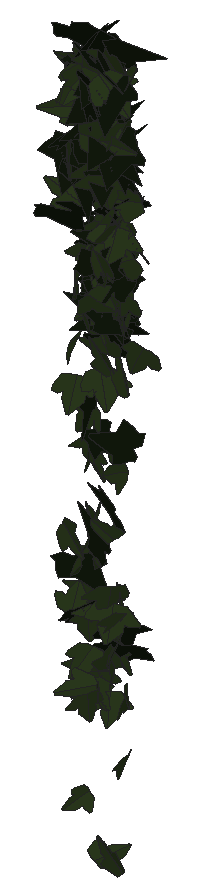
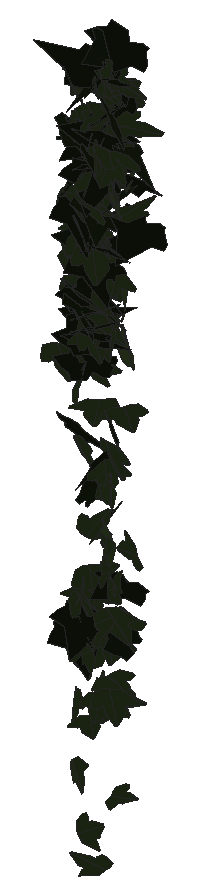
# SketchUp Ruby script. Lengths in inches.
U = 1.inch
M = Sketchup.active_model
def pt(a) = Geom::Point3d.new(a.map { |v| v * U })
def face(e, loops, mat)
  f = e.add_face(loops[0].map { |a| pt(a) })
  loops[1..].each { |l| e.add_face(l.map { |a| pt(a) }).erase! }
  f.material = f.back_material = mat if mat
  f
end
# faces: each face lists its corners as indices into pts; further lists are holes
def faces(e, pts, list, mat = nil) = list.each { |f| face(e, (f[0].is_a?(Array) ? f : [f]).map { |l| l.map { |i| pts[i] } }, mat) }
# xy, xz, yz: faces in a plane at the given z, y or x. An outline is a flat list of corners, or four numbers for a rectangle; further outlines are holes
def ring(l) = l.size == 4 ? [[l[0], l[1]], [l[2], l[1]], [l[2], l[3]], [l[0], l[3]]] : l.each_slice(2).to_a
def flat(e, list, mat, &to3) = list.each { |f| face(e, (f[0].is_a?(Array) ? f : [f]).map { |l| ring(l).map { |u, v| to3.(u, v) } }, mat) }
def xy(e, z, list, mat = nil) = flat(e, list, mat) { |x, y| [x, y, z] }
def xz(e, y, list, mat = nil) = flat(e, list, mat) { |x, z| [x, y, z] }
def yz(e, x, list, mat = nil) = flat(e, list, mat) { |y, z| [x, y, z] }
def lines(e, pts, list) = list.each { |a, b| e.add_line(pt(pts[a]), pt(pts[b])) }
# prism: a flat outline (further loops are holes) pulled along v
def prism(e, loops, v, mat = nil)
  f = face(e, loops, mat); d = Geom::Vector3d.new(v.map { |x| x * U })
  f.pushpull(f.normal.samedirection?(d) ? d.length : -d.length)
end
def box(e, o, s, mat = nil) = prism(e, [[o, [o[0] + s[0], o[1], o[2]], [o[0] + s[0], o[1] + s[1], o[2]], [o[0], o[1] + s[1], o[2]]]], [0, 0, s[2]], mat)
def at(x, y, z, deg = 0) = Geom::Transformation.translation(pt([x, y, z])) * Geom::Transformation.rotation(ORIGIN, Z_AXIS, deg.degrees)
def axes(o, x, y, z) = Geom::Transformation.new([*x, 0, *y, 0, *z, 0, *pt(o).to_a, 1])
def part(name) = M.definitions.add(name)
# library, detail: a bought-in or finely detailed component or shape, given as its bounding box
def library(name, o, s) = part(name).tap { |d| box(d.entities, o, s) }
def detail(e, o, s) = box(e.add_group.entities, o, s)
def put(e, d, t, mat = nil) = e.add_instance(d, t).tap { |i| i.material = mat if mat }
def group(e, t, mat = nil) = e.add_group.tap { |g| g.transformation = t; g.material = mat if mat }.entities
root = M.entities
M.materials.add("1026 AP 7946 SUNNY SIDE UP").color = [254, 231, 186]
M.materials.add("efeu1").color = [18, 25, 13]
M.materials.add("efeu2").color = [43, 57, 29]
c1 = part("ivyleaf_10")
p = [[0,0.5,-0.03],[-0.0625,2.02,-0.43],[-0.19,2.01,-0.46],[-0.54,1.05,-0.29],[-0.52,0.625,-0.18],[-0.83,0.76,-0.28],
  [-1.16,0.64,-0.33],[-1.15,0.33,-0.24],[-0.77,-0.39,0.02],[-0.3,-0.51,0.16],[0.04,-0.48,0.23],[-0.02,2.01,-0.4375],
  [-0.06,2.01,-0.43],[0.04,-0.49,0.23],[0.67,-0.49,0.14],[1.38,0.36,-0.2],[1.375,0.51,-0.24],[0.81,0.65,-0.19],
  [0.62,0.59,-0.15],[0.6,1.09,-0.28],[0.5,1.23,-0.31]]
faces(c1.entities,p,[[0,1,2,3,4,5,6,7,8,9,10],[11,12,0,13,14,15,16,17,18,19,20]],"efeu2")
c2 = part("ivyleaf_9")
p = [[1.54,2.16,1.25],[1.36,2.04,1.19],[-0.21,0.99,0.68],[-0.71,1.11,0.82],[-0.85,0.86,0.67],[-0.8,0.17,0.21],
  [-0.9,-0.01,0.1],[-0.67,-0.16,-0.02],[-0.08,-0.08,-0.05],[-0.03,-0.6,-0.4],[0.65,-0.88,-0.66],[0.83,-0.6,-0.49],
  [1.29,-0.42,-0.43],[1.8125,-0.07,-0.26],[1.21,0.44,0.15]]
faces(c2.entities,p,[[0,1,2,3,4,5,6,7,8,9,10,11,12,13,14]],"efeu1")
put(root,c1,axes([144.45,212.06,261.74],[0.01803,-0.18534,-0.18854],[0.09388,-0.17538,0.18688],[-0.39747,-0.04983,0.03559]),"1026 AP 7946 SUNNY SIDE UP")
put(root,c1,axes([144.87,211.93,255.18],[-0.1348,-0.22159,-0.03975],[0.06097,0.02477,-0.24305],[0.34804,-0.09016,0.02718]),"1026 AP 7946 SUNNY SIDE UP")
put(root,c1,axes([144.71,212.06,253.23],[0.088,0.07575,-0.18545],[-0.14235,-0.15637,-0.09747],[-0.27281,0.10602,-0.00896]),"1026 AP 7946 SUNNY SIDE UP")
put(root,c1,axes([144.34,212.09,265.43],[-0.07276,0.14566,-0.23472],[0.08159,-0.22293,-0.15841],[-0.41843,-0.0688,0.00993]),"1026 AP 7946 SUNNY SIDE UP")
put(root,c2,axes([145.21,212.11,266.96],[-0.32431,-0.1331,-0.196],[0.34711,-0.03636,-0.22143],[0.10998,-0.27772,0.1209]),"1026 AP 7946 SUNNY SIDE UP")
put(root,c1,axes([145.13,211.92,263.67],[-0.315,0.15747,0.02528],[-0.04992,-0.00227,-0.2616],[-0.24536,-0.20171,0.02078]),"1026 AP 7946 SUNNY SIDE UP")
put(root,c2,axes([145.16,211.98,258.11],[-0.04449,-0.23121,0.13442],[0.04104,0.12949,0.24055],[-0.41646,0.03746,0.00935]),"1026 AP 7946 SUNNY SIDE UP")
put(root,c1,axes([145.04,211.86,262.92],[-0.1515,-0.15169,-0.19123],[0.17748,0.14673,-0.18389],[0.33135,-0.14795,0.01106]),"1026 AP 7946 SUNNY SIDE UP")
put(root,c1,axes([145.5,211.92,252.2],[-0.20704,0.08706,-0.17581],[-0.21304,0.10493,0.16299],[0.21396,0.18873,-0.00784]),"1026 AP 7946 SUNNY SIDE UP")
put(root,c1,axes([144.92,211.94,265.875],[-0.00116,-0.00938,0.2927],[0.41626,0.10365,0.00484],[-0.16311,0.26459,0.01027]),"1026 AP 7946 SUNNY SIDE UP")
put(root,c2,axes([145.27,212.12,258.8],[0.15451,-0.24106,0.03262],[0.00824,0.03771,0.26769],[-0.3825,-0.09656,0.01894]),"1026 AP 7946 SUNNY SIDE UP")
put(root,c1,axes([145.125,211.91,263.71],[-0.02194,0.23657,0.10266],[-0.00865,0.09815,-0.24356],[-0.40272,-0.01499,-0.00036]),"1026 AP 7946 SUNNY SIDE UP")
put(root,c1,axes([144.45,212.09,264.51],[0.02544,0.20991,0.15199],[-0.10758,-0.13774,0.21053],[0.38771,-0.05199,0.04845]),"1026 AP 7946 SUNNY SIDE UP")
put(root,c1,axes([144.6,212.15,266.86],[0.14605,0.16517,-0.21623],[-0.18426,-0.1756,-0.19593],[-0.37868,0.14915,0.01194]),"1026 AP 7946 SUNNY SIDE UP")
put(root,c1,axes([144.54,212.14,266.875],[0.17303,0.19063,-0.17859],[-0.11346,-0.15939,-0.22727],[-0.39015,0.1309,-0.01312]),"1026 AP 7946 SUNNY SIDE UP")
put(root,c2,axes([145.09,211.89,263.4],[-0.12994,-0.02228,0.24889],[0.33848,0.11129,0.08703],[-0.17642,0.22994,-0.01633]),"1026 AP 7946 SUNNY SIDE UP")
put(root,c1,axes([145.28,212.06,256.92],[0.36629,0.11595,-0.02087],[-0.01282,-0.03038,-0.26715],[-0.18482,0.23191,-0.02284]),"1026 AP 7946 SUNNY SIDE UP")
put(root,c2,axes([144.22,211.9,264.32],[0.34278,0.1723,-0.00282],[0.01511,-0.01813,-0.28561],[-0.27057,0.21727,-0.01952]),"1026 AP 7946 SUNNY SIDE UP")
put(root,c1,axes([145.26,212.05,257.3],[-0.21369,-0.23241,0.00403],[0.00829,-0.00914,-0.27725],[0.36544,-0.13569,0.00865]),"1026 AP 7946 SUNNY SIDE UP")
put(root,c2,axes([144.92,211.9,266.41],[0.04695,-0.02726,0.29068],[-0.11428,0.27366,0.03674],[-0.43108,-0.07551,0.02192]),"1026 AP 7946 SUNNY SIDE UP")
put(root,c1,axes([144.24,212.14,258.07],[0.13555,-0.0311,0.23828],[0.33648,-0.08832,-0.09484],[0.14711,0.23067,-0.00262]),"1026 AP 7946 SUNNY SIDE UP")
put(root,c2,axes([145.24,212.2,266.0625],[-0.34855,-0.16205,-0.01746],[0.04188,-0.00937,-0.28191],[0.2526,-0.22205,0.02264]),"1026 AP 7946 SUNNY SIDE UP")
put(root,c1,axes([145.42,212.13,256.8125],[-0.07764,-0.24735,0.06803],[-0.02721,-0.06531,-0.26019],[0.40221,-0.05216,-0.00447]),"1026 AP 7946 SUNNY SIDE UP")
put(root,c1,axes([144.4,212.24,262.9],[-0.04091,0.05186,-0.26232],[0.0678,-0.25179,-0.05878],[-0.40339,-0.04758,0.01672]),"1026 AP 7946 SUNNY SIDE UP")
put(root,c1,axes([144.57,212.18,266.27],[0.12976,0.00512,-0.27205],[-0.37496,-0.11758,-0.0798],[-0.17867,0.25047,-0.03011]),"1026 AP 7946 SUNNY SIDE UP")
put(root,c2,axes([144.71,212.125,267.34],[0.28113,-0.21539,0.05224],[0.08571,-0.02193,-0.28712],[0.33768,0.18489,0.02938]),"1026 AP 7946 SUNNY SIDE UP")
put(root,c1,axes([145.22,211.98,266.99],[0.17671,0.24407,0.12792],[0.11107,0.10229,-0.27549],[-0.41499,0.1313,-0.01927]),"1026 AP 7946 SUNNY SIDE UP")
put(root,c1,axes([145.52,212.01,259.7],[0.16452,-0.14291,-0.17497],[-0.18773,0.12099,-0.18081],[0.29307,0.15773,-0.0176]),"1026 AP 7946 SUNNY SIDE UP")
put(root,c2,axes([144.5625,212.04,265.84],[-0.20079,0.24005,-0.04224],[0.00496,-0.04619,-0.27971],[-0.38325,-0.12636,0.01851]),"1026 AP 7946 SUNNY SIDE UP")
put(root,c1,axes([145.11,212.08,265.06],[-0.32834,-0.16825,-0.03101],[0.05736,0.00102,-0.27532],[0.2623,-0.21083,0.02139]),"1026 AP 7946 SUNNY SIDE UP")
put(root,c1,axes([145.14,212.2,258.25],[-0.15622,-0.12955,-0.14412],[-0.16373,-0.0943,0.16647],[-0.25013,0.14263,-0.01896]),"1026 AP 7946 SUNNY SIDE UP")
put(root,c2,axes([145.26,212.24,265.77],[-0.28645,-0.19422,-0.06174],[0.11708,0.00957,-0.27003],[0.29684,-0.1912,0.04693]),"1026 AP 7946 SUNNY SIDE UP")
put(root,c2,axes([144.42,212.29,264.92],[0.04612,-0.27459,0.10193],[0.01391,-0.10013,-0.28507],[0.45957,0.03059,-0.0016]),"1026 AP 7946 SUNNY SIDE UP")
put(root,c1,axes([145.375,212.19,266.09],[-0.01546,-0.29313,0.06983],[0.03207,-0.06998,-0.3017],[0.47259,-0.00484,0.02276]),"1026 AP 7946 SUNNY SIDE UP")
put(root,c1,axes([145.31,212.18,256.375],[0.18709,-0.22729,0.04707],[0.03074,-0.04279,-0.26454],[0.36365,0.12055,-0.00185]),"1026 AP 7946 SUNNY SIDE UP")
put(root,c1,axes([144.63,212.26,255.18],[-0.1137,0.00947,0.23017],[-0.13325,-0.2184,-0.02],[0.32531,-0.08615,0.07225]),"1026 AP 7946 SUNNY SIDE UP")
put(root,c2,axes([144.78,212.34,266.36],[-0.17899,-0.16344,0.19714],[-0.11589,-0.18023,-0.20381],[0.37953,-0.13211,0.03074]),"1026 AP 7946 SUNNY SIDE UP")
put(root,c1,axes([145.19,212.07,265.95],[0.07529,0.08139,0.30112],[-0.47619,0.00452,0.04992],[0.01345,-0.2957,0.08178]),"1026 AP 7946 SUNNY SIDE UP")
put(root,c2,axes([144.58,212.05,266.91],[0.42803,-0.06141,-0.13887],[-0.21558,0.00042,-0.28615],[0.08688,0.30361,-0.02585]),"1026 AP 7946 SUNNY SIDE UP")
put(root,c2,axes([144.375,212.25,265.36],[-0.34713,-0.11976,-0.11273],[0.19364,-0.00511,-0.25177],[0.16495,-0.24604,0.05832]),"1026 AP 7946 SUNNY SIDE UP")
put(root,c2,axes([144.99,212.07,265.83],[-0.07772,-0.11834,-0.26902],[0.19136,0.23051,-0.13034],[0.40711,-0.13095,0.00991]),"1026 AP 7946 SUNNY SIDE UP")
put(root,c2,axes([145.03,212.3125,266.1],[-0.01931,-0.02639,-0.26721],[-0.01289,-0.25935,0.02608],[-0.40952,0.0094,0.01178]),"1026 AP 7946 SUNNY SIDE UP")
put(root,c1,axes([145.1,212.3,255.68],[-0.05123,0.02836,0.25146],[0.23785,-0.19153,0.04263],[0.3042,0.15453,0.00901]),"1026 AP 7946 SUNNY SIDE UP")
put(root,c2,axes([144.49,212.03,267.78],[0.41426,0.11758,-0.00252],[0.01035,-0.02238,-0.29639],[-0.18465,0.26253,-0.02228]),"1026 AP 7946 SUNNY SIDE UP")
put(root,c1,axes([145.24,212.19,264.03],[0.3744,0.09825,-0.03775],[-0.04011,-0.03533,-0.26454],[-0.16026,0.23839,-0.02199]),"1026 AP 7946 SUNNY SIDE UP")
put(root,c1,axes([144.77,212.1,267.06],[0.04095,-0.0314,-0.28786],[-0.38408,0.13611,-0.03844],[0.21843,0.24521,-0.01363]),"1026 AP 7946 SUNNY SIDE UP")
put(root,c2,axes([144.86,212.3,265.38],[-0.19112,-0.24931,-0.07187],[0.08085,0.0507,-0.28443],[0.39836,-0.1299,0.02325]),"1026 AP 7946 SUNNY SIDE UP")
put(root,c1,axes([144.92,212.21,265.18],[-0.21788,-0.25791,-0.00189],[0.0244,-0.00792,-0.30113],[0.4048,-0.13834,0.01714]),"1026 AP 7946 SUNNY SIDE UP")
put(root,c1,axes([145.42,212.1875,262.89],[-0.35227,0.02531,0.08134],[-0.1277,-0.0232,-0.23028],[-0.02519,-0.23636,0.0299]),"1026 AP 7946 SUNNY SIDE UP")
put(root,c1,axes([144.8,212.34,255.27],[0.02106,-0.08763,-0.19104],[0.04436,-0.18278,0.09026],[-0.31873,-0.03123,-0.00006]),"1026 AP 7946 SUNNY SIDE UP")
put(root,c2,axes([145.28,212.06,262.98],[-0.3796,0.11924,-0.02877],[-0.02554,0.0315,0.27673],[0.19111,0.24105,-0.02016]),"1026 AP 7946 SUNNY SIDE UP")
put(root,c1,axes([145.27,212.22,262.72],[-0.14967,0.22471,-0.06088],[0.02468,-0.05888,-0.25161],[-0.36504,-0.09612,0.00795]),"1026 AP 7946 SUNNY SIDE UP")
put(root,c2,axes([144.86,212.38,267.09],[-0.33121,-0.18708,-0.02494],[0.08661,-0.02789,-0.28434],[0.28347,-0.21006,0.05774]),"1026 AP 7946 SUNNY SIDE UP")
put(root,c2,axes([145.55,212.1875,265.95],[-0.19466,0.25977,-0.08402],[0.03907,-0.08007,-0.29668],[-0.42704,-0.12574,0.01116]),"1026 AP 7946 SUNNY SIDE UP")
put(root,c1,axes([144.38,212.16,256.66],[0.28428,0.09421,-0.05119],[0.05584,0.04007,0.20938],[0.15831,-0.18331,0.01805]),"1026 AP 7946 SUNNY SIDE UP")
put(root,c1,axes([144.34,212.27,260.86],[0.26605,0.18015,-0.06878],[-0.05309,-0.06107,-0.2544],[-0.29797,0.17174,-0.01608]),"1026 AP 7946 SUNNY SIDE UP")
put(root,c1,axes([145.11,212.26,255.79],[-0.14736,-0.23233,-0.00077],[-0.01318,0.004,0.25793],[-0.36508,0.09363,-0.009]),"1026 AP 7946 SUNNY SIDE UP")
put(root,c2,axes([145.59,212.1875,260.1],[-0.23486,0.11899,0.15627],[-0.20768,0.07545,-0.19539],[-0.21968,-0.19854,0.01765]),"1026 AP 7946 SUNNY SIDE UP")
put(root,c1,axes([145.14,212.3,264.05],[0.02192,-0.28309,0.03968],[0.00196,-0.04011,-0.29222],[0.44958,0.01398,-0.00066]),"1026 AP 7946 SUNNY SIDE UP")
put(root,c2,axes([145.26,212.32,262.35],[-0.06913,0.03542,0.26603],[-0.40687,-0.03572,-0.04058],[0.04661,-0.2593,0.04036]),"1026 AP 7946 SUNNY SIDE UP")
put(root,c1,axes([144.71,212.36,267.18],[-0.08,-0.23749,0.10208],[-0.01748,-0.10025,-0.25061],[0.40507,-0.05123,0.00934]),"1026 AP 7946 SUNNY SIDE UP")
put(root,c1,axes([144.93,212.3125,263.48],[0.37461,0.1275,-0.0471],[-0.05222,-0.0362,-0.27809],[-0.20687,0.24001,-0.01509]),"1026 AP 7946 SUNNY SIDE UP")
put(root,c2,axes([144.37,212.25,257.53],[-0.09035,-0.08544,-0.2263],[0.2236,0.16712,-0.10454],[0.29467,-0.15301,0.00994]),"1026 AP 7946 SUNNY SIDE UP")
put(root,c1,axes([144.54,212.39,265.14],[0.15601,-0.11197,0.2319],[0.32621,-0.10141,-0.14635],[0.2249,0.22477,0.05141]),"1026 AP 7946 SUNNY SIDE UP")
put(root,c2,axes([145.07,212.35,265.77],[-0.23415,0.13725,-0.16435],[0.15446,-0.12857,-0.20816],[-0.29369,-0.17704,0.02156]),"1026 AP 7946 SUNNY SIDE UP")
put(root,c1,axes([145.22,212.34,257.18],[-0.08052,0.16283,-0.11666],[0.03608,-0.11227,-0.17622],[-0.31062,-0.05525,0.00978]),"1026 AP 7946 SUNNY SIDE UP")
put(root,c1,axes([145.32,212.42,262.68],[-0.06326,0.15986,0.21155],[0.09919,-0.19465,0.16845],[0.39583,0.07433,-0.0084]),"1026 AP 7946 SUNNY SIDE UP")
put(root,c1,axes([144.44,212.46,257.46],[-0.00047,-0.0311,0.23673],[0.09639,-0.22181,-0.03212],[0.35193,0.06071,0.00911]),"1026 AP 7946 SUNNY SIDE UP")
put(root,c2,axes([145.38,212.23,256.21],[0.18876,0.17539,-0.13406],[-0.14858,-0.09342,-0.21838],[-0.31064,0.15126,0.02299]),"1026 AP 7946 SUNNY SIDE UP")
put(root,c1,axes([145.04,212.22,261.43],[-0.20874,0.09554,-0.16977],[-0.19585,0.1093,0.16874],[0.22758,0.18169,-0.0105]),"1026 AP 7946 SUNNY SIDE UP")
put(root,c2,axes([144.79,212.0625,267.59],[-0.11961,0.16373,-0.22113],[-0.1512,0.19299,0.18708],[0.3979,0.12255,0.00461]),"1026 AP 7946 SUNNY SIDE UP")
put(root,c1,axes([144.74,212.39,262.72],[0.27737,-0.12132,0.13499],[0.16752,-0.07752,-0.22099],[0.22633,0.20605,-0.00187]),"1026 AP 7946 SUNNY SIDE UP")
put(root,c2,axes([144.29,212.23,256.4],[0.15595,0.22004,-0.0028],[-0.02326,0.01101,0.24802],[0.34526,-0.09864,0.01797]),"1026 AP 7946 SUNNY SIDE UP")
put(root,c1,axes([144.59,212.2,262.35],[-0.13101,0.18597,0.13553],[-0.11093,0.11095,-0.20864],[-0.33957,-0.108,0.01587]),"1026 AP 7946 SUNNY SIDE UP")
put(root,c2,axes([144.54,212.43,260.6],[-0.1959,0.03669,-0.21702],[0.29814,-0.09429,-0.13285],[-0.15615,-0.22605,0.01861]),"1026 AP 7946 SUNNY SIDE UP")
put(root,c2,axes([145.25,212.2,256.52],[0.22526,0.21164,-0.00606],[0.01364,-0.01441,-0.2629],[-0.33269,0.14271,-0.01488]),"1026 AP 7946 SUNNY SIDE UP")
put(root,c1,axes([144.49,212.46,257.5625],[0.01264,-0.03648,-0.2218],[0.1719,-0.18559,0.03555],[-0.29687,-0.10902,0.01114]),"1026 AP 7946 SUNNY SIDE UP")
put(root,c2,axes([145.21,212.26,265.34],[0.27686,-0.12512,-0.16591],[-0.18616,0.10938,-0.22123],[0.26002,0.21153,0.01827]),"1026 AP 7946 SUNNY SIDE UP")
put(root,c1,axes([144.89,212.24,265.81],[-0.0009,-0.22201,-0.17373],[0.01471,0.16727,-0.22762],[0.43694,-0.00609,0.0073]),"1026 AP 7946 SUNNY SIDE UP")
put(root,c2,axes([144.96,212.46,263.83],[-0.34187,-0.1527,-0.0625],[0.09703,0.01583,-0.27268],[0.23891,-0.22494,0.0213]),"1026 AP 7946 SUNNY SIDE UP")
put(root,c1,axes([144.66,212.1875,266.34],[0.15756,0.10775,0.243],[0.17727,0.20891,-0.14681],[-0.36624,0.14747,0.03348]),"1026 AP 7946 SUNNY SIDE UP")
put(root,c1,axes([144.51,212.42,255.71],[0.22448,0.14896,-0.1351],[-0.13669,-0.09945,-0.21308],[-0.28152,0.16707,-0.00427]),"1026 AP 7946 SUNNY SIDE UP")
put(root,c1,axes([145.41,212.42,267.03],[0.18537,-0.23932,0.0513],[0.01612,-0.0519,-0.27479],[0.38446,0.11757,-0.01321]),"1026 AP 7946 SUNNY SIDE UP")
put(root,c1,axes([144.74,212.36,266.13],[-0.15406,0.22876,-0.07993],[0.03693,-0.07572,-0.25669],[-0.37869,-0.10045,0.00749]),"1026 AP 7946 SUNNY SIDE UP")
put(root,c1,axes([144.57,212.35,256.41],[-0.28681,-0.11,-0.00011],[0.01364,-0.01538,-0.21877],[0.17243,-0.18175,0.01712]),"1026 AP 7946 SUNNY SIDE UP")
put(root,c1,axes([144.4,212.51,265.11],[0.15301,-0.16876,0.21123],[0.18569,-0.16923,-0.20128],[0.37531,0.15253,0.01347]),"1026 AP 7946 SUNNY SIDE UP")
put(root,c1,axes([144.625,212.33,255.16],[-0.21522,-0.16312,-0.1],[0.16473,0.03358,-0.21214],[0.248,-0.16386,0.05413]),"1026 AP 7946 SUNNY SIDE UP")
put(root,c1,axes([145.37,212.38,263.51],[-0.25768,0.01909,0.19953],[-0.29732,-0.075,-0.15773],[0.07174,-0.24229,0.06299]),"1026 AP 7946 SUNNY SIDE UP")
put(root,c1,axes([144.92,212.375,264.32],[0.26676,-0.22068,-0.05817],[-0.0697,0.03549,-0.28622],[0.35084,0.17484,-0.01263]),"1026 AP 7946 SUNNY SIDE UP")
put(root,c1,axes([144.69,212.35,263.43],[-0.4162,-0.07677,-0.0186],[0.03667,-0.0174,-0.28302],[0.11829,-0.2647,0.02231]),"1026 AP 7946 SUNNY SIDE UP")
put(root,c1,axes([144.7,212.27,258.2],[0.152,-0.15659,0.15189],[-0.10304,0.13354,0.19001],[-0.32312,-0.11625,0.01086]),"1026 AP 7946 SUNNY SIDE UP")
put(root,c1,axes([144.55,212.41,256.9],[-0.28252,-0.07896,0.12796],[-0.16434,-0.07057,-0.20165],[0.16381,-0.20699,0.0184]),"1026 AP 7946 SUNNY SIDE UP")
put(root,c1,axes([145.09,212.33,267.06],[-0.34187,0.08805,-0.1842],[-0.24317,0.09355,0.24106],[0.19881,0.26583,-0.0219]),"1026 AP 7946 SUNNY SIDE UP")
put(root,c1,axes([145.41,212.4,264.64],[0.09064,0.0079,-0.26738],[-0.40837,0.00297,-0.0593],[0.00186,0.2659,0.01016]),"1026 AP 7946 SUNNY SIDE UP")
put(root,c1,axes([145.07,212.41,256.03],[-0.22642,0.09139,-0.12882],[0.15322,-0.08016,-0.1757],[-0.19015,-0.17342,0.01182]),"1026 AP 7946 SUNNY SIDE UP")
put(root,c2,axes([144.97,212.2,265.89],[0.03628,0.0122,0.28893],[0.30886,0.20025,-0.02446],[-0.31521,0.19762,0.00929]),"1026 AP 7946 SUNNY SIDE UP")
put(root,c1,axes([144.87,212.41,261.63],[-0.35359,0.00293,-0.05951],[-0.08985,0.02519,0.23054],[0.0143,0.23081,-0.02304]),"1026 AP 7946 SUNNY SIDE UP")
put(root,c1,axes([144.83,212.55,262.46],[-0.18593,-0.109,0.22079],[-0.15558,-0.19635,-0.15981],[0.34554,-0.14706,0.04685]),"1026 AP 7946 SUNNY SIDE UP")
put(root,c1,axes([144.9,212.4,265.15],[-0.21883,-0.20418,-0.05025],[0.06152,0.03086,-0.25393],[0.32388,-0.14382,0.01428]),"1026 AP 7946 SUNNY SIDE UP")
put(root,c2,axes([144.9,212.5625,266.125],[-0.39564,-0.11176,0.01156],[-0.00125,-0.0273,-0.28266],[0.17671,-0.25041,0.02388]),"1026 AP 7946 SUNNY SIDE UP")
put(root,c1,axes([144.6,212.41,265.65],[-0.41869,0.10358,-0.04608],[0.04973,-0.04308,-0.29314],[-0.17067,-0.26664,0.02762]),"1026 AP 7946 SUNNY SIDE UP")
put(root,c1,axes([145.09,212.46,263.96],[-0.21201,-0.21897,0.01388],[0.01074,-0.02145,-0.26446],[0.34492,-0.13393,0.01677]),"1026 AP 7946 SUNNY SIDE UP")
put(root,c2,axes([144.98,212.53,264.06],[0.2291,-0.17995,0.10294],[0.08829,-0.08433,-0.23886],[0.31219,0.15591,-0.00799]),"1026 AP 7946 SUNNY SIDE UP")
put(root,c1,axes([145.29,212.4375,263.61],[-0.22791,0.01276,-0.19367],[-0.29086,0.03604,0.14959],[0.05705,0.23469,-0.01103]),"1026 AP 7946 SUNNY SIDE UP")
put(root,c1,axes([144.52,212.62,257.85],[0.0151,0.059,-0.22865],[-0.05583,-0.21943,-0.06287],[-0.35729,0.03678,0.00016]),"1026 AP 7946 SUNNY SIDE UP")
put(root,c2,axes([144.91,212.38,265.28],[0.29109,0.14587,-0.09158],[-0.08993,-0.07188,-0.24238],[-0.25382,0.19275,-0.01915]),"1026 AP 7946 SUNNY SIDE UP")
put(root,c1,axes([144.9,212.55,266.05],[-0.11716,0.17993,-0.16351],[0.05669,-0.15699,-0.20042],[-0.37407,-0.08015,0.02084]),"1026 AP 7946 SUNNY SIDE UP")
put(root,c1,axes([144.82,212.36,251.95],[0.17041,0.04924,-0.18797],[0.24278,0.09878,0.12233],[0.1721,-0.1881,0.01356]),"1026 AP 7946 SUNNY SIDE UP")
put(root,c1,axes([144.44,212.51,265.84],[0.43987,0.03401,-0.00136],[0.00267,-0.02643,-0.28919],[-0.05347,0.2785,-0.02561]),"1026 AP 7946 SUNNY SIDE UP")
put(root,c2,axes([145.09,212.59,263.09],[0.00619,0.03619,-0.2502],[-0.06157,-0.23991,-0.03885],[-0.38149,0.0393,0.00221]),"1026 AP 7946 SUNNY SIDE UP")
put(root,c1,axes([145.11,212.43,263.96],[0.30015,-0.17421,0.0458],[-0.02263,0.05126,0.265],[-0.28219,-0.18941,0.02747]),"1026 AP 7946 SUNNY SIDE UP")
put(root,c2,axes([144.88,212.52,262.1],[0.40746,0.04031,-0.00401],[-0.00032,0.02793,0.26883],[0.06371,-0.25766,0.02696]),"1026 AP 7946 SUNNY SIDE UP")
put(root,c1,axes([145.2,212.49,262.54],[0.28046,-0.17912,-0.06639],[-0.08135,0.03793,-0.26001],[0.2875,0.18547,-0.00881]),"1026 AP 7946 SUNNY SIDE UP")
put(root,c1,axes([144.59,212.49,259.77],[-0.20777,-0.20508,-0.00191],[0.023,-0.00861,-0.25077],[0.32164,-0.13186,0.0167]),"1026 AP 7946 SUNNY SIDE UP")
put(root,c2,axes([144.85,212.45,263.65],[0.18453,0.1716,-0.15585],[-0.10917,-0.13644,-0.21434],[-0.34381,0.13542,-0.01559]),"1026 AP 7946 SUNNY SIDE UP")
put(root,c2,axes([145.21,212.43,262.95],[-0.24256,0.20458,0.09452],[-0.17307,0.02641,-0.25438],[-0.3063,-0.17693,0.06888]),"1026 AP 7946 SUNNY SIDE UP")
put(root,c1,axes([144.46,212.51,255.42],[-0.29012,-0.14204,0.03905],[-0.0333,-0.03581,-0.23958],[0.22909,-0.18509,0.01463]),"1026 AP 7946 SUNNY SIDE UP")
put(root,c2,axes([145.19,212.39,264.51],[0.11787,0.25065,-0.06861],[-0.02556,-0.06613,-0.26989],[-0.40758,0.07663,-0.00292]),"1026 AP 7946 SUNNY SIDE UP")
put(root,c1,axes([144.97,212.44,262.96],[-0.30439,0.08789,-0.18264],[-0.24441,0.08707,0.21921],[0.19368,0.248,-0.01042]),"1026 AP 7946 SUNNY SIDE UP")
put(root,c1,axes([145.28,212.4,255.11],[0.05764,-0.17605,-0.16548],[0.00375,0.16178,-0.1823],[0.37366,0.02554,0.02736]),"1026 AP 7946 SUNNY SIDE UP")
put(root,c2,axes([144.84,212.55,261.6],[0.38787,0.05895,0.0657],[-0.10604,0.01063,0.26005],[0.08543,-0.25448,0.02451]),"1026 AP 7946 SUNNY SIDE UP")
put(root,c1,axes([144.83,212.53,263.86],[-0.29218,-0.19948,0.01902],[0.00286,-0.02839,-0.28021],[0.31516,-0.18468,0.02017]),"1026 AP 7946 SUNNY SIDE UP")
put(root,c2,axes([144.67,212.6,262.8],[0.01408,-0.24961,-0.03405],[0.08845,0.03284,-0.25035],[0.38561,0.00158,0.05867]),"1026 AP 7946 SUNNY SIDE UP")
put(root,c1,axes([144.85,212.51,262.31],[0.15788,0.24844,-0.03609],[-0.06555,-0.02221,-0.27444],[-0.38934,0.10448,0.03157]),"1026 AP 7946 SUNNY SIDE UP")
put(root,c1,axes([144.49,212.55,259.4375],[-0.22215,0.10114,-0.11958],[0.11638,-0.0944,-0.17721],[-0.21305,-0.15702,0.02789]),"1026 AP 7946 SUNNY SIDE UP")
put(root,c1,axes([144.83,212.57,262.34],[-0.12978,-0.24875,0.05335],[-0.00411,-0.0551,-0.2699],[0.39996,-0.08128,0.01454]),"1026 AP 7946 SUNNY SIDE UP")
put(root,c2,axes([144.82,212.47,267.19],[0.26674,-0.17755,-0.13591],[-0.14528,0.09278,-0.25242],[0.31498,0.19316,-0.00133]),"1026 AP 7946 SUNNY SIDE UP")
put(root,c1,axes([144.41,212.63,259.32],[0.0066,-0.16638,-0.13791],[0.00145,-0.13294,0.17067],[-0.33486,-0.00385,-0.00198]),"1026 AP 7946 SUNNY SIDE UP")
put(root,c1,axes([145.26,212.39,261.08],[-0.12926,0.28375,-0.14643],[-0.05568,0.13938,0.30512],[0.49704,0.08941,-0.0039]),"1026 AP 7946 SUNNY SIDE UP")
put(root,c1,axes([144.7,212.52,260.98],[0.25805,0.20704,0.00786],[0.03309,-0.00848,-0.27129],[-0.32402,0.16402,-0.02145]),"1026 AP 7946 SUNNY SIDE UP")
put(root,c2,axes([145.04,212.67,262.24],[-0.34654,-0.06861,0.11886],[-0.15405,-0.07048,-0.23559],[0.14506,-0.23876,0.03375]),"1026 AP 7946 SUNNY SIDE UP")
put(root,c2,axes([144.74,212.62,262.47],[-0.0342,-0.24406,-0.04559],[0.08223,0.03754,-0.24731],[0.38086,-0.03002,0.0493]),"1026 AP 7946 SUNNY SIDE UP")
put(root,c2,axes([144.875,212.5,267.34],[0.28901,0.06057,-0.18891],[0.23371,0.11798,0.19395],[0.19468,-0.23155,0.04761]),"1026 AP 7946 SUNNY SIDE UP")
put(root,c1,axes([144.68,212.52,255.28],[-0.25737,-0.11399,-0.0371],[0.06085,0.0061,-0.20472],[0.17753,-0.16735,0.01638]),"1026 AP 7946 SUNNY SIDE UP")
put(root,c2,axes([145.16,212.43,262.86],[-0.04007,0.24708,0.00765],[0.00322,0.00627,-0.25584],[-0.38861,-0.02543,-0.00291]),"1026 AP 7946 SUNNY SIDE UP")
put(root,c1,axes([144.84,212.57,254.89],[0.18898,0.19425,-0.04353],[-0.03247,-0.0382,-0.23553],[-0.31126,0.12192,-0.00186]),"1026 AP 7946 SUNNY SIDE UP")
put(root,c2,axes([144.27,212.54,266.37],[-0.04478,0.22826,0.18074],[0.02383,-0.17356,0.2359],[0.45081,0.03185,0.00548]),"1026 AP 7946 SUNNY SIDE UP")
put(root,c1,axes([144.93,212.6,264.74],[0.36383,-0.0241,0.09755],[0.14477,-0.02879,-0.23913],[0.05208,0.2484,-0.01676]),"1026 AP 7946 SUNNY SIDE UP")
put(root,c1,axes([144.55,212.41,256.7],[-0.00329,0.17379,0.15877],[-0.01411,0.15296,-0.17807],[-0.36395,-0.0075,0.00547]),"1026 AP 7946 SUNNY SIDE UP")
put(root,c2,axes([144.91,212.37,264.61],[0.04725,0.23983,0.10979],[-0.03838,0.10801,-0.24582],[-0.41001,0.01752,0.03567]),"1026 AP 7946 SUNNY SIDE UP")
put(root,c1,axes([144.43,212.56,258.3125],[-0.20203,0.17188,-0.05219],[0.03265,-0.04884,-0.221],[-0.28031,-0.12957,0.01188]),"1026 AP 7946 SUNNY SIDE UP")
put(root,c1,axes([145.54,212.56,261.72],[-0.34643,-0.00818,0.09435],[-0.14062,-0.0367,-0.22511],[0.03391,-0.23577,0.03036]),"1026 AP 7946 SUNNY SIDE UP")
put(root,c1,axes([145.16,212.58,253.85],[0.03456,-0.20946,-0.00067],[-0.00277,-0.00073,-0.21696],[0.32934,0.02197,-0.00176]),"1026 AP 7946 SUNNY SIDE UP")
put(root,c2,axes([144.62,212.46,259.96],[0.14485,-0.11809,-0.20266],[-0.13735,0.1772,-0.1512],[0.33264,0.12459,0.02582]),"1026 AP 7946 SUNNY SIDE UP")
put(root,c1,axes([144.41,212.57,260.24],[0.32659,-0.12542,-0.06488],[-0.07303,0.04337,-0.24936],[0.20771,0.21245,0.01434]),"1026 AP 7946 SUNNY SIDE UP")
